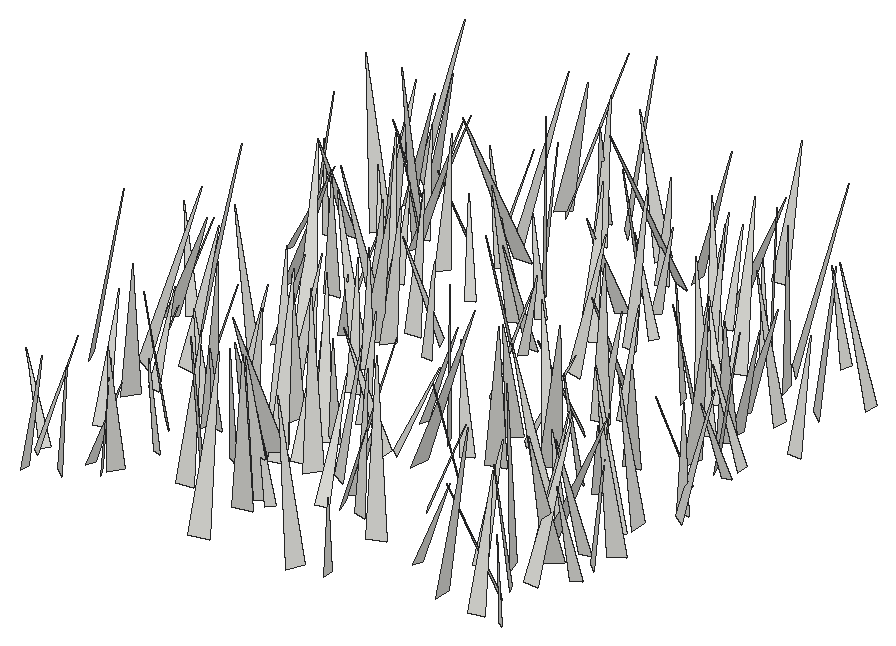
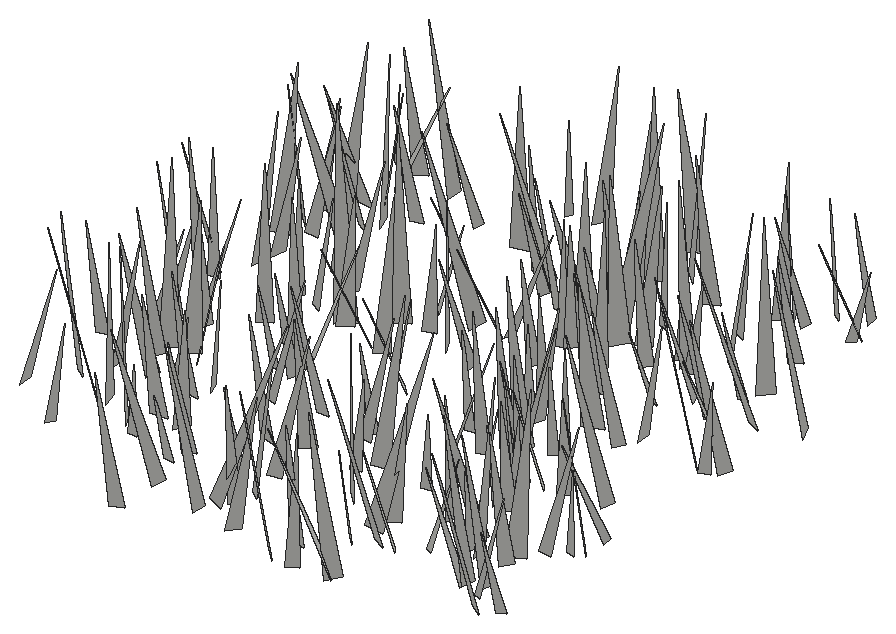
# SketchUp Ruby script. Lengths in inches.
U = 1.inch
M = Sketchup.active_model
def pt(a) = Geom::Point3d.new(a.map { |v| v * U })
def face(e, loops, mat)
  f = e.add_face(loops[0].map { |a| pt(a) })
  loops[1..].each { |l| e.add_face(l.map { |a| pt(a) }).erase! }
  f.material = f.back_material = mat if mat
  f
end
# faces: each face lists its corners as indices into pts; further lists are holes
def faces(e, pts, list, mat = nil) = list.each { |f| face(e, (f[0].is_a?(Array) ? f : [f]).map { |l| l.map { |i| pts[i] } }, mat) }
# xy, xz, yz: faces in a plane at the given z, y or x. An outline is a flat list of corners, or four numbers for a rectangle; further outlines are holes
def ring(l) = l.size == 4 ? [[l[0], l[1]], [l[2], l[1]], [l[2], l[3]], [l[0], l[3]]] : l.each_slice(2).to_a
def flat(e, list, mat, &to3) = list.each { |f| face(e, (f[0].is_a?(Array) ? f : [f]).map { |l| ring(l).map { |u, v| to3.(u, v) } }, mat) }
def xy(e, z, list, mat = nil) = flat(e, list, mat) { |x, y| [x, y, z] }
def xz(e, y, list, mat = nil) = flat(e, list, mat) { |x, z| [x, y, z] }
def yz(e, x, list, mat = nil) = flat(e, list, mat) { |y, z| [x, y, z] }
def lines(e, pts, list) = list.each { |a, b| e.add_line(pt(pts[a]), pt(pts[b])) }
# prism: a flat outline (further loops are holes) pulled along v
def prism(e, loops, v, mat = nil)
  f = face(e, loops, mat); d = Geom::Vector3d.new(v.map { |x| x * U })
  f.pushpull(f.normal.samedirection?(d) ? d.length : -d.length)
end
def box(e, o, s, mat = nil) = prism(e, [[o, [o[0] + s[0], o[1], o[2]], [o[0] + s[0], o[1] + s[1], o[2]], [o[0], o[1] + s[1], o[2]]]], [0, 0, s[2]], mat)
def at(x, y, z, deg = 0) = Geom::Transformation.translation(pt([x, y, z])) * Geom::Transformation.rotation(ORIGIN, Z_AXIS, deg.degrees)
def axes(o, x, y, z) = Geom::Transformation.new([*x, 0, *y, 0, *z, 0, *pt(o).to_a, 1])
def part(name) = M.definitions.add(name)
# library, detail: a bought-in or finely detailed component or shape, given as its bounding box
def library(name, o, s) = part(name).tap { |d| box(d.entities, o, s) }
def detail(e, o, s) = box(e.add_group.entities, o, s)
def put(e, d, t, mat = nil) = e.add_instance(d, t).tap { |i| i.material = mat if mat }
def group(e, t, mat = nil) = e.add_group.tap { |g| g.transformation = t; g.material = mat if mat }.entities
root = M.entities
c1 = part("fur_instance\#9")
p = [[0.8125,0,1.79],[0.67,-0.02,1.48],[0,-0.11,0],[0,0.11,0]]
faces(c1.entities,p,[[0,1,2,3]])
put(root,c1,axes([499.63,421.45,-21.66],[6.18065,2.99725,1.89028],[2.99834,-6.44896,0.42186],[-1.88855,-0.42956,6.85609]))
put(root,c1,axes([500.26,456.0625,-21.66],[-0.72601,3.76819,0.7458],[3.80081,0.81458,-0.41575],[0.55615,-0.64789,3.8149]))
put(root,c1,axes([501.63,430.7,-21.66],[-2.18486,3.79279,1.02862],[3.92891,2.13324,0.47945],[0.08359,-1.13179,4.35074]))
put(root,c1,axes([501.8,446.09,-21.66],[0.50374,3.60666,1.32904],[3.78488,-0.69911,0.46265],[-0.67011,-1.23747,3.61216]))
put(root,c1,axes([501.12,445.19,-21.66],[4.60486,4.04407,1.88978],[4.30358,-4.74303,-0.33665],[-1.18533,-1.50984,6.1193]))
put(root,c1,axes([501.34,428.43,-21.66],[4.04394,2.43918,0.42992],[2.39305,-4.06014,0.52577],[-0.63852,0.23141,4.69325]))
put(root,c1,axes([500.875,442.96,-21.66],[4.1398,0.29454,0.02134],[0.28882,-4.10074,0.57065],[-0.06159,0.56772,4.11084]))
put(root,c1,axes([500.51,429.625,-21.66],[5.28357,-2.5058,0.04843],[-2.504,-5.27298,0.35108],[0.10676,0.33794,5.83712]))
put(root,c1,axes([503.16,455.23,-21.66],[-1.78915,-3.44674,0.35763],[-3.41457,1.82215,0.479],[0.59044,0.09337,3.85378]))
put(root,c1,axes([503.31,447.18,-21.66],[-0.2394,-4.99537,0.47277],[-5.01072,0.21306,-0.28607],[-0.26442,0.48521,4.99291]))
put(root,c1,axes([501.99,456.89,-21.66],[3.861,5.57007,1.34937],[5.71182,-3.87341,-0.35436],[-0.47072,-1.31331,6.76812]))
put(root,c1,axes([504.5625,448.95,-21.66],[-4.39266,5.33205,2.64396],[5.82364,4.52851,0.54275],[1.2274,-2.40386,6.88706]))
put(root,c1,axes([505.53,408.68,-21.66],[-3.05082,2.35934,0.28628],[2.37608,3.01778,0.45074],[-0.05159,-0.53147,3.83025]))
put(root,c1,axes([502.97,429.98,-21.66],[5.7382,5.20942,1.87337],[5.41352,-5.84467,-0.3291],[-1.15821,-1.50876,7.74318]))
put(root,c1,axes([503.29,422.85,-21.66],[3.5873,6.66463,1.07182],[6.75002,-3.55215,-0.50434],[-0.05834,-1.18311,7.55193]))
put(root,c1,axes([503.45,453.67,-21.66],[5.71322,-0.96407,0.62556],[-0.92485,-5.73993,-0.39936],[-0.68221,-0.29224,5.7802]))
put(root,c1,axes([504.38,450.26,-21.66],[3.71133,-3.4553,1.19556],[-3.62183,-3.7076,0.52772],[-0.50083,1.20708,5.04327]))
put(root,c1,axes([505.4,407.75,-21.66],[2.99735,3.72962,0.28981],[3.68324,-3.00724,0.60693],[-0.65404,0.15682,4.74613]))
put(root,c1,axes([504.83,454.17,-21.66],[6.44965,-0.53992,1.19924],[-0.48241,-6.55498,-0.35669],[-1.22351,-0.26161,6.46237]))
put(root,c1,axes([506.6875,413.67,-21.66],[-1.85743,4.94831,0.92273],[4.99711,1.93095,-0.29602],[0.60509,-0.75691,5.27714]))
put(root,c1,axes([506.23,420.38,-21.66],[-0.0874,4.08723,0.80677],[4.1529,0.14964,-0.30818],[0.33125,-0.79758,4.07653]))
put(root,c1,axes([506.19,405.4,-21.66],[4.45017,0.43948,1.54669],[0.28501,-4.6951,0.51402],[-1.58245,0.39027,4.44218]))
put(root,c1,axes([505.49,418.73,-21.66],[5.14782,-4.26055,1.16689],[-4.27581,-5.25589,-0.32723],[-1.10966,0.4872,6.67423]))
put(root,c1,axes([504.15,438.8,-21.66],[6.51578,-0.90085,0.09034],[-0.89347,-6.50413,-0.41604],[-0.1463,-0.39981,6.56459]))
put(root,c1,axes([506.85,450.32,-21.66],[-6.68895,-1.28776,2.75903],[-1.15,7.23488,0.5888],[2.81923,-0.10417,6.78629]))
put(root,c1,axes([504.95,454.59,-21.66],[4.62251,0.92588,0.22465],[0.9419,-4.60847,-0.38752],[-0.14333,-0.42437,4.69837]))
put(root,c1,axes([506.24,424.2,-21.66],[-0.03084,5.75903,1.17934],[5.85206,0.14189,-0.53988],[0.55736,-1.17118,5.73375]))
put(root,c1,axes([508.36,429.35,-21.66],[-5.56537,0.35389,1.01892],[0.25962,5.63719,-0.53984],[1.04691,0.48332,5.55042]))
put(root,c1,axes([507.75,449.98,-21.66],[-3.18277,2.93848,0.48438],[2.88307,3.21784,-0.5768],[0.74643,0.10079,4.29324]))
put(root,c1,axes([507.6,439.44,-21.66],[1.5026,-5.2869,1.47769],[-5.48951,-1.44343,0.41772],[0.01326,1.53554,5.48039]))
put(root,c1,axes([508.65,448.72,-21.66],[-3.91635,-3.27614,1.36892],[-3.24396,4.13005,0.60351],[1.44353,0.39293,5.07017]))
put(root,c1,axes([509.24,443.92,-21.66],[3.60121,-2.60608,3.3834],[-3.59297,-4.24118,0.55747],[-2.30861,2.53545,4.41017]))
put(root,c1,axes([508.61,406.51,-21.66],[2.85129,3.39796,1.84964],[3.79237,-2.9092,-0.50161],[-0.76499,-1.75715,4.40731]))
put(root,c1,axes([510.41,441.83,-21.66],[-3.8761,2.85036,0.12124],[2.83481,3.87102,-0.37744],[0.32105,0.23257,4.79648]))
put(root,c1,axes([510.11,452.15,-21.66],[-1.91573,-3.10975,0.18965],[-3.07242,1.92263,0.49017],[0.51647,-0.09744,3.61944]))
put(root,c1,axes([510.35,416.87,-21.66],[-3.95359,-4.39819,1.62013],[-4.4402,4.19331,0.54823],[1.50116,0.81969,5.8885]))
put(root,c1,axes([509.02,422.57,-21.66],[4.30125,1.72732,0.68489],[1.69718,-4.35514,0.32517],[-0.75649,0.05042,4.6237]))
put(root,c1,axes([510.15,442.01,-21.66],[3.4021,4.35261,1.87369],[4.47593,-3.70904,0.48912],[-1.55627,-1.15238,5.50275]))
put(root,c1,axes([508.04,448.61,-21.66],[6.4862,-0.82849,0.61771],[-0.87391,-6.49276,0.46816],[-0.55158,0.54452,6.52212]))
put(root,c1,axes([510.38,443.73,-21.66],[-2.95191,2.4359,0.97471],[2.3622,3.10602,-0.60836],[1.1418,-0.12828,3.77853]))
put(root,c1,axes([509.4,439.62,-21.66],[3.16954,2.48643,0.53995],[2.54162,-3.13416,-0.48689],[-0.1185,-0.71733,3.99891]))
put(root,c1,axes([512.21,430.4,-21.66],[-3.14428,7.71271,0.49149],[7.72648,3.12546,0.38342],[-0.17032,-0.59964,8.32018]))
put(root,c1,axes([509.08,431.34,-21.66],[4.36325,-2.68491,0.18726],[-2.69098,-4.34538,0.39756],[0.04948,0.43666,5.1077]))
put(root,c1,axes([511.69,419.69,-21.66],[-3.05036,2.77962,1.08054],[2.93347,3.07501,0.37088],[0.53722,-1.00823,4.11016]))
put(root,c1,axes([511.12,424.8,-21.66],[1.03899,3.82207,0.22987],[3.79032,-1.06041,0.49963],[-0.54276,-0.08876,3.92914]))
put(root,c1,axes([509.55,408.9375,-21.66],[4.16125,-1.09144,0.28201],[-1.11074,-4.15389,0.31328],[-0.19241,0.37504,4.29058]))
put(root,c1,axes([512.47,438.875,-21.66],[-6.25427,-0.78477,1.30734],[-0.71032,6.38344,0.43371],[1.34924,-0.27711,6.28838]))
put(root,c1,axes([510.92,408.51,-21.66],[4.15437,2.45212,1.76514],[2.75663,-4.30471,-0.50784],[-1.23677,-1.35794,4.79727]))
put(root,c1,axes([511.65,447.32,-21.66],[4.3952,-2.19196,2.60814],[-2.70598,-4.83259,0.49862],[-2.06997,1.6632,4.88608]))
put(root,c1,axes([512.28,413.18,-21.66],[0.90627,3.33198,1.59944],[3.57947,-1.20149,0.47479],[-0.9207,-1.39138,3.42023]))
put(root,c1,axes([511.11,440.0625,-21.66],[3.01124,-3.84874,1.35887],[-4.04465,-3.04041,0.35153],[-0.54781,1.29229,4.87409]))
put(root,c1,axes([511.59,409.36,-21.66],[4.45698,-3.93649,1.376],[-3.92382,-4.64074,-0.56675],[-1.41173,0.47074,5.91941]))
put(root,c1,axes([512,435.36,-21.66],[1.97582,-3.11414,0.08334],[-3.10691,-1.9626,0.3224],[0.22782,0.24287,3.67393]))
put(root,c1,axes([512.125,453.625,-21.66],[3.35941,2.47012,0.56366],[2.52325,-3.34641,-0.37364],[-0.22894,-0.63632,4.15301]))
put(root,c1,axes([512.65,418.83,-21.66],[7.01983,-0.71592,2.31882],[-0.6287,-7.39114,-0.37866],[-2.34397,-0.1616,7.04608]))
put(root,c1,axes([515.92,432.38,-21.66],[-6.2227,2.39174,0.32304],[2.36421,6.22042,-0.51348],[0.48507,0.36431,6.64671]))
put(root,c1,axes([513.51,418.64,-21.66],[0.0585,-4.06465,0.78718],[-4.11626,0.02739,0.44734],[0.44434,0.78888,4.04038]))
put(root,c1,axes([514.78,450.38,-21.66],[2.55776,-3.86723,2.22173],[-4.13899,-3.01226,-0.47827],[-1.66143,1.55064,4.61182]))
put(root,c1,axes([513.74,436.98,-21.66],[3.88682,0.49651,1.01606],[0.42112,-4.01087,0.34905],[-1.04955,0.22945,3.90283]))
put(root,c1,axes([513.02,459.66,-21.66],[5.25974,-3.61511,1.15521],[-3.73911,-5.27428,0.51907],[-0.65007,1.0869,6.36116]))
put(root,c1,axes([515.29,452.08,-21.66],[-0.22294,-7.81188,0.28991],[-7.80547,0.20653,-0.4373],[-0.42917,0.30182,7.80282]))
put(root,c1,axes([513.73,453.51,-21.66],[3.6487,6.36792,1.23917],[6.47764,-3.65398,-0.29593],[-0.35515,-1.22351,7.3332]))
put(root,c1,axes([513.47,459.41,-21.66],[5.3948,4.35682,0.5893],[4.31887,-5.42625,0.57994],[-0.82254,0.08385,6.9101]))
put(root,c1,axes([514.63,426.04,-21.66],[0.44242,5.64748,1.29703],[5.78226,-0.34572,-0.46699],[0.37666,-1.32609,5.6455]))
put(root,c1,axes([516.04,445.05,-21.66],[-1.47936,3.73163,0.54523],[3.76451,1.42617,0.45319],[-0.22551,-0.67216,3.98851]))
put(root,c1,axes([515.53,454.49,-21.66],[2.40724,3.27999,1.19788],[3.2967,-2.61439,0.53362],[-1.15108,-0.62824,4.03341]))
put(root,c1,axes([514.82,420.93,-21.66],[3.66382,-3.28739,1.57998],[-3.52995,-3.75957,0.36325],[-0.918,1.33625,4.90903]))
put(root,c1,axes([514.3125,435.91,-21.66],[4.31409,-4.88001,1.43702],[-5.06352,-4.30068,0.59646],[-0.49016,1.47666,6.48614]))
put(root,c1,axes([515.33,436.38,-21.66],[-4.36102,2.95909,2.58691],[3.11538,4.95832,-0.41976],[2.39639,-1.06094,5.25343]))
put(root,c1,axes([516.44,432.55,-21.66],[-4.17339,1.81444,1.20525],[1.74242,4.34394,-0.50613],[1.30721,0.0026,4.52253]))
put(root,c1,axes([515.98,438.43,-21.66],[-1.18817,5.57554,2.26119],[5.96275,1.39894,-0.31626],[0.80332,-2.13721,5.69196]))
put(root,c1,axes([518.3,438.93,-21.66],[-4.34148,-1.68145,0.56308],[-1.64517,4.37512,0.38015],[0.66161,-0.1544,4.64018]))
put(root,c1,axes([516.375,460.26,-21.66],[1.54796,-4.76639,0.70367],[-4.81569,-1.50748,0.38266],[0.1508,0.78667,4.99682]))
put(root,c1,axes([517.9375,429.02,-21.66],[-0.91047,5.0165,1.03079],[5.11456,0.83694,0.44447],[-0.2628,-1.09133,5.07905]))
put(root,c1,axes([516.94,410.7,-21.66],[-1.46748,5.77462,2.34569],[6.13429,1.76496,-0.50731],[1.10405,-2.13089,5.93652]))
put(root,c1,axes([517.21,423.36,-21.66],[5.69628,-2.00129,2.37758],[-1.98509,-6.1627,-0.4314],[-2.39112,0.34864,6.02217]))
put(root,c1,axes([517.49,415.62,-21.66],[-2.05605,-4.2865,1.82271],[-4.5186,2.31917,0.35698],[1.13077,1.47345,4.74068]))
put(root,c1,axes([516.99,418.56,-21.66],[3.45501,-4.88886,0.26504],[-4.85303,-3.46254,-0.60598],[-0.64754,-0.13474,5.95575]))
put(root,c1,axes([518.24,457.41,-21.66],[-0.17119,5.69768,1.30234],[5.83131,0.07859,0.42267],[-0.39436,-1.31119,5.68456]))
put(root,c1,axes([518.46,419.55,-21.66],[-5.59489,5.13542,2.2708],[5.22691,5.9344,-0.54239],[2.05147,-1.11455,7.57503]))
put(root,c1,axes([518.95,423.23,-21.66],[-3.597,-0.64897,1.74683],[-0.97146,3.89365,-0.55385],[1.59023,0.91068,3.61287]))
put(root,c1,axes([518.89,436.38,-21.66],[0.06663,3.86387,1.64805],[4.18879,0.06273,-0.31643],[0.31563,-1.6482,3.85147]))
put(root,c1,axes([519.43,449.48,-21.66],[4.46233,4.90899,2.88894],[5.22756,-4.98695,0.39938],[-2.26203,-1.84084,6.62202]))
put(root,c1,axes([518.79,459.83,-21.66],[4.76999,5.26227,1.90717],[5.37132,-5.00824,0.38463],[-1.57405,-1.14351,7.09199]))
put(root,c1,axes([520.09,417.51,-21.66],[-1.2461,7.24945,1.28302],[7.36015,1.19663,0.38699],[-0.1701,-1.32928,7.34558]))
put(root,c1,axes([520.79,422.01,-21.66],[-4.49131,4.50007,0.95246],[4.50728,4.57122,-0.34355],[0.91773,-0.42777,6.34858]))
put(root,c1,axes([520.58,408.52,-21.66],[3.92843,5.06138,3.38638],[5.5366,-4.64662,0.52215],[-2.53598,-2.30413,6.38572]))
put(root,c1,axes([519.85,418,-21.66],[2.00321,-7.73932,0.37509],[-7.71802,-2.02729,-0.61059],[-0.68548,0.20889,7.97102]))
put(root,c1,axes([520.65,444.66,-21.66],[2.01145,-6.31603,1.30369],[-6.40118,-2.12156,-0.40211],[-0.78536,1.11557,6.61638]))
put(root,c1,axes([521.14,418.45,-21.66],[-1.57636,3.66287,0.67143],[3.67727,1.64614,-0.34684],[0.58749,-0.47537,3.97256]))
put(root,c1,axes([521.75,446.1,-21.66],[-1.38179,3.78074,1.32931],[4.00762,1.30133,0.46468],[-0.00636,-1.40818,3.99842]))
put(root,c1,axes([521.38,425.9,-21.66],[2.89571,-2.97183,2.13904],[-3.49598,-3.05481,0.48854],[-1.08874,1.90494,4.12046]))
put(root,c1,axes([521.46,422.47,-21.66],[0.51611,-4.80053,1.29544],[-4.96034,-0.40702,0.46794],[0.34389,1.33374,4.80546]))
put(root,c1,axes([523.24,458.54,-21.66],[-5.24229,2.67543,1.59997],[2.88849,5.34612,0.52444],[1.17239,-1.20849,5.86212]))
put(root,c1,axes([523.01,418.05,-21.66],[-6.12251,3.37612,2.03098],[3.42132,6.417,-0.35327],[1.95387,-0.65732,6.98272]))
put(root,c1,axes([522.54,405.29,-21.66],[-2.30774,6.81626,2.09214],[7.04491,2.51871,-0.43516],[1.09893,-1.8327,7.18315]))
put(root,c1,axes([522.82,412.42,-21.66],[2.11565,-6.08651,1.80009],[-6.2822,-2.27872,-0.32139],[-0.90548,1.58863,6.43571]))
put(root,c1,axes([523.21,441.02,-21.66],[-3.17607,-4.40082,1.193],[-4.40846,3.33508,0.56622],[1.16445,0.62283,5.3976]))
put(root,c1,axes([523.72,412.16,-21.66],[1.42768,-3.34431,1.65268],[-3.54003,-1.77266,-0.52903],[-1.17641,1.27565,3.59761]))
put(root,c1,axes([522.42,410.53,-21.66],[2.16747,-6.96935,1.82134],[-7.20329,-2.08612,0.58967],[0.04123,1.91397,7.27476]))
put(root,c1,axes([524.07,442.1875,-21.66],[-0.19346,-4.85951,0.89963],[-4.92735,0.1202,-0.41034],[-0.38132,0.91231,4.84602]))
put(root,c1,axes([525.48,423.48,-21.66],[-5.10669,0.68056,0.36828],[0.71376,5.09217,0.48729],[0.29888,-0.53268,5.12875]))
put(root,c1,axes([524.06,441.12,-21.66],[3.08181,-1.73974,0.98019],[-1.88437,-3.1302,0.36886],[-0.66077,0.81254,3.51969]))
put(root,c1,axes([525.2,453.6,-21.66],[-3.25628,-4.53556,1.56998],[-4.60157,3.48952,0.53691],[1.36443,0.94415,5.55755]))
put(root,c1,axes([526.71,456.3,-21.66],[-3.06964,-6.81398,0.3454],[-6.81954,3.05272,-0.38339],[-0.20825,0.47214,7.46364]))
put(root,c1,axes([525.09,418.38,-21.66],[2.3418,4.95634,1.60959],[5.19702,-2.35112,-0.32146],[-0.38351,-1.59595,5.4723]))
put(root,c1,axes([525.81,450.5625,-21.66],[1.38462,-5.25865,0.1546],[-5.22749,-1.39323,-0.57157],[-0.5921,0.00308,5.40776]))
put(root,c1,axes([524.69,428.875,-21.66],[4.46137,-0.22154,0.62784],[-0.29219,-4.4737,0.49769],[-0.59824,0.53291,4.43905]))
put(root,c1,axes([525.53,455.53,-21.66],[2.1664,-3.98299,1.68795],[-4.30586,-2.16689,0.41322],[-0.41582,1.68731,4.51516]))
put(root,c1,axes([526.5625,445.68,-21.66],[-2.92394,5.35838,1.35906],[5.44647,3.05552,-0.32925],[0.94614,-1.02969,6.09534]))
put(root,c1,axes([526.66,414.47,-21.66],[-2.17484,4.53028,0.06229],[4.50087,2.16823,-0.54601],[0.51907,0.1805,4.99552]))
put(root,c1,axes([526.32,434.56,-21.66],[3.1839,3.43631,0.24845],[3.39454,-3.18669,0.57383],[-0.5891,0.20968,4.64932]))
put(root,c1,axes([525.89,423.99,-21.66],[2.47782,3.1575,0.0552],[3.13992,-2.45577,-0.47176],[0.33732,-0.3344,3.98583]))
put(root,c1,axes([527.96,427.76,-21.66],[5.01686,3.02729,2.73746],[3.17963,-5.61852,0.38618],[-2.55892,-1.04628,5.84673]))
put(root,c1,axes([527.83,452.02,-21.66],[3.18405,-1.52738,1.26596],[-1.78098,-3.25535,0.55182],[-0.87386,1.06936,3.48806]))
put(root,c1,axes([527.39,417.14,-21.66],[3.65064,-1.60023,0.53489],[-1.66152,-3.63138,0.47591],[-0.29361,0.65299,3.95745]))
put(root,c1,axes([530.08,448.92,-21.66],[-3.96056,0.86775,0.15545],[0.85071,3.94968,-0.37345],[0.23119,0.33194,4.03727]))
put(root,c1,axes([527.08,457.82,-21.66],[6.44978,-0.00096,0.92482],[0.04605,-6.50733,-0.32793],[-0.92367,-0.33115,6.44144]))
put(root,c1,axes([529.59,446.68,-21.66],[0.8824,6.11345,1.2337],[6.18895,-1.01221,0.58924],[-0.77016,-1.12963,6.14863]))
put(root,c1,axes([527.76,415.58,-21.66],[6.78168,2.91502,1.19431],[2.8839,-6.88568,0.43057],[-1.26762,-0.07012,7.36906]))
put(root,c1,axes([528.84,441.17,-21.66],[0.94432,5.62245,1.27282],[5.76049,-0.87093,-0.42662],[0.22085,-1.32412,5.68522]))
put(root,c1,axes([529.69,415.08,-21.66],[1.56528,5.39191,1.82425],[5.61252,-1.77733,0.43748],[-0.9488,-1.61836,5.59744]))
put(root,c1,axes([530.79,406.22,-21.66],[-6.02179,2.8816,2.13168],[3.11245,6.27078,0.31555],[1.77772,-1.21792,6.66828]))
put(root,c1,axes([530.41,426.75,-21.66],[1.59272,-3.9303,2.28796],[-4.37909,-1.9795,-0.352],[-1.22702,1.96293,4.22612]))
put(root,c1,axes([528.25,423.85,-21.66],[7.76844,-0.71206,0.72464],[-0.74639,-7.79129,0.34557],[-0.68922,0.41169,7.79335]))
put(root,c1,axes([531.84,423.93,-21.66],[-3.00946,-2.45302,0.73779],[-2.54129,3.00205,-0.38468],[0.32167,0.76736,3.86344]))
put(root,c1,axes([531.17,431.29,-21.66],[3.50702,-4.68842,0.88051],[-4.69288,-3.58696,-0.4079],[-0.85643,0.45629,5.84073]))
put(root,c1,axes([532.91,413,-21.66],[-2.11891,6.73628,2.3501],[7.12334,2.13432,0.30482],[0.39806,-2.33612,7.05509]))
put(root,c1,axes([531.97,461.18,-21.66],[-1.06035,5.5551,1.84187],[5.77115,1.30347,-0.60889],[0.97234,-1.67863,5.62252]))
put(root,c1,axes([532.98,441.95,-21.66],[-1.82356,-4.42835,0.39133],[-4.41286,1.85435,0.42054],[0.53859,0.19978,4.77062]))
put(root,c1,axes([533.375,453.39,-21.66],[-0.09668,3.9627,0.07364],[3.92699,0.08582,0.53775],[-0.5359,-0.08606,3.92724]))
put(root,c1,axes([532.85,451.67,-21.66],[-1.4542,4.67664,1.33998],[4.76533,1.65076,-0.58976],[0.97884,-1.08869,4.86188]))
put(root,c1,axes([533.3,406.875,-21.66],[3.51099,-0.42801,1.09439],[-0.295,-3.65871,-0.48452],[-1.13748,-0.37227,3.50364]))
put(root,c1,axes([534.71,434.94,-21.66],[-3.28468,-3.33783,0.1825],[-3.30088,3.27904,0.56182],[0.52783,-0.26523,4.64915]))
put(root,c1,axes([533.04,418.79,-21.66],[3.15167,2.15202,0.19961],[2.1362,-3.1554,0.29004],[-0.32814,0.12762,3.80527]))
put(root,c1,axes([532.47,430.95,-21.66],[3.00056,3.161,0.00616],[3.13284,-2.97269,-0.58633],[0.42105,-0.40809,4.31874]))
put(root,c1,axes([531.8,456.5625,-21.66],[5.92157,-1.3609,0.111],[-1.36516,-5.91048,0.36315],[-0.02664,0.3788,6.06507]))
put(root,c1,axes([532.87,426.97,-21.66],[3.4393,-6.56896,1.063],[-6.65437,-3.3911,0.57422],[0.02233,1.20797,7.39258]))
put(root,c1,axes([535.6,449.12,-21.66],[-5.07407,3.61415,0.85454],[3.5922,5.14344,-0.42375],[0.94256,-0.14624,6.2152]))
put(root,c1,axes([533.98,438.07,-21.66],[3.92282,-1.4058,1.44453],[-1.66907,-4.03753,0.60333],[-1.1301,1.0833,4.1232]))
put(root,c1,axes([535.75,429.85,-21.66],[2.97491,-4.25566,3.74848],[-5.0806,-3.88069,-0.37363],[-2.51977,2.80026,5.17891]))
put(root,c1,axes([534.66,436.96,-21.66],[-1.49682,6.02983,3.22428],[6.74332,1.8484,-0.32627],[1.1325,-3.03643,6.20426]))
put(root,c1,axes([535.79,437.98,-21.66],[0.78964,4.34465,0.57519],[4.335,-0.86018,0.54605],[-0.64386,-0.46311,4.38193]))
put(root,c1,axes([537.44,443.09,-21.66],[-4.30965,-1.39305,1.63599],[-1.58025,4.5392,-0.29767],[1.45598,0.80324,4.51941]))
put(root,c1,axes([538.45,425.7,-21.66],[-6.00997,1.04438,1.22572],[1.13938,6.10462,0.38513],[1.13796,-0.59647,6.08787]))
put(root,c1,axes([537.79,452.15,-21.66],[-0.46969,3.55211,0.73396],[3.59032,0.35011,0.60316],[-0.51554,-0.79795,3.53189]))
put(root,c1,axes([538.04,448.76,-21.66],[-1.0825,6.58238,0.66021],[6.6005,1.02978,0.55528],[-0.44383,-0.73975,6.64764]))
put(root,c1,axes([538.19,444.93,-21.66],[-0.0106,6.43156,0.96228],[6.47441,-0.07994,0.60561],[-0.61077,-0.95901,6.403]))
put(root,c1,axes([536,429.49,-21.66],[5.23004,-6.31048,0.45418],[-6.32662,-5.22094,0.31214],[-0.04891,0.54893,8.19012]))
put(root,c1,axes([539.91,444.24,-21.66],[-2.40389,3.30252,0.08348],[3.28439,2.37806,0.4999],[-0.35549,-0.36124,4.05406]))
put(root,c1,axes([539.24,428.98,-21.66],[1.51862,3.68557,2.40948],[4.21899,-1.94756,0.31991],[-1.2606,-2.07817,3.97332]))
put(root,c1,axes([537.43,412.21,-21.66],[4.04534,-0.8517,0.30361],[-0.87788,-4.03293,0.38361],[-0.21657,0.43867,4.11619]))
put(root,c1,axes([539.35,450.86,-21.66],[5.6621,3.46946,2.68851],[3.90579,-5.98471,-0.5026],[-2.00251,-1.86297,6.62147]))
put(root,c1,axes([540.9375,440.56,-21.66],[-4.28874,-2.62611,1.19653],[-2.76089,4.3576,-0.33198],[0.84,0.91449,5.01792]))
put(root,c1,axes([541.32,423.95,-21.66],[1.53479,-3.08573,1.52348],[-3.30012,-1.79268,-0.30636],[-0.97569,1.2095,3.43271]))
put(root,c1,axes([541.95,440.05,-21.66],[-4.3858,5.26104,2.02142],[5.54364,4.48874,0.34523],[1.01623,-1.78118,6.84066]))
put(root,c1,axes([541.33,414.58,-21.66],[-0.63443,5.02312,1.44392],[5.17666,0.80438,-0.52377],[0.72032,-1.3566,5.03586]))
put(root,c1,axes([540.72,433.05,-21.66],[2.46673,-5.38252,0.46134],[-5.39282,-2.42347,0.55987],[0.31917,0.65147,5.89431]))
put(root,c1,axes([542.3,449.09,-21.66],[5.88559,1.89129,2.87248],[1.95642,-6.52369,0.2867],[-2.82853,-0.57687,6.17535]))
put(root,c1,axes([541.33,428.39,-21.66],[1.84889,-3.8875,0.07331],[-3.87281,-1.83403,0.41727],[0.34554,0.24513,4.2845]))
put(root,c1,axes([541.73,409.71,-21.66],[7.00703,0.38351,2.14023],[0.30488,-7.32356,0.31416],[-2.15283,0.21111,7.01048]))
put(root,c1,axes([543.16,416.17,-21.66],[-6.66859,-2.01923,2.71074],[-2.32845,7.09045,-0.44648],[2.45024,1.24248,6.95328]))
put(root,c1,axes([541.03,451.59,-21.66],[5.81873,5.70667,1.51485],[5.84557,-5.86726,-0.35074],[-0.83073,-1.31442,8.14252]))
put(root,c1,axes([543.62,454.43,-21.66],[-3.82053,1.38738,1.41647],[1.59253,3.97908,0.39802],[1.18113,-0.87734,4.0451]))
put(root,c1,axes([545.35,412.03,-21.66],[-3.79986,-3.34827,0.10157],[-3.34083,3.7767,-0.4853],[-0.24505,0.43103,5.04126]))
put(root,c1,axes([545.16,444.76,-21.66],[-5.94659,0.26274,1.16381],[0.1992,6.05181,-0.34844],[1.17635,0.30341,5.94219]))
put(root,c1,axes([542.13,444.33,-21.66],[5.3173,-1.56529,0.48292],[-1.59322,-5.32309,0.28875],[-0.38078,0.41424,5.53538]))
put(root,c1,axes([545.08,413.49,-21.66],[-4.18009,-2.38384,1.39005],[-2.61185,4.23208,-0.59649],[0.8906,1.22265,4.77494]))
put(root,c1,axes([543.9,417.67,-21.66],[2.83544,5.2975,1.05869],[5.3487,-2.92083,0.29014],[-0.75876,-0.79328,6.00159]))
put(root,c1,axes([546.26,424.5625,-21.66],[-6.22467,1.67352,0.58559],[1.62437,6.23957,-0.56507],[0.71064,0.39649,6.42089]))
put(root,c1,axes([545.46,434,-21.66],[-2.21382,-3.77344,0.32599],[-3.76288,2.23425,0.30817],[0.43109,0.1241,4.36404]))
put(root,c1,axes([543.75,436.35,-21.66],[6.97924,-1.80721,1.76653],[-1.77915,-7.19853,-0.33521],[-1.79479,0.10824,7.20163]))
put(root,c1,axes([543.86,440.26,-21.66],[3.44417,-6.15496,0.43731],[-6.17002,-3.42915,0.33004],[0.07525,0.54268,7.04535]))
put(root,c1,axes([543.71,441.61,-21.66],[5.53978,-0.90724,0.62547],[-0.85463,-5.56113,-0.49688],[-0.69563,-0.39269,5.59154]))
put(root,c1,axes([545.49,408.95,-21.66],[-2.00411,5.21831,1.67163],[5.38658,2.20263,-0.41796],[1.00489,-1.39973,5.57427]))
put(root,c1,axes([546.15,420.79,-21.66],[0.08099,-5.17118,1.20761],[-5.27072,-0.22549,-0.61212],[-0.64729,1.18913,5.13546]))
put(root,c1,axes([545.11,418.52,-21.66],[3.26606,-6.16963,0.62937],[-6.14796,-3.31446,-0.58694],[-0.81426,0.27855,6.95607]))
put(root,c1,axes([543.04,420.59,-21.66],[6.75875,-1.16964,0.00047],[-1.16859,-6.75255,0.29358],[0.0496,0.28936,6.85293]))
put(root,c1,axes([545.83,414.93,-21.66],[0.77683,6.56918,0.32302],[6.56801,-0.79193,0.30978],[-0.34589,-0.28401,6.60769]))
put(root,c1,axes([547.17,437.86,-21.66],[-4.29082,0.07848,0.62907],[0.12494,4.3243,0.31276],[0.62151,-0.32753,4.28013]))
put(root,c1,axes([546.57,426.47,-21.66],[5.59524,-0.57904,3.08549],[-0.36766,-6.38318,-0.53118],[-3.11775,-0.28642,5.59999]))
put(root,c1,axes([545.68,436.68,-21.66],[5.68987,2.39384,1.65752],[2.61602,-5.80047,-0.60296],[-1.2784,-1.21517,6.14342]))
put(root,c1,axes([547.16,436.09,-21.66],[0.58704,-3.79537,0.45103],[-3.78334,-0.64184,-0.47675],[-0.5428,0.36891,3.81079]))
put(root,c1,axes([548.85,450.76,-21.66],[-5.68888,-0.08485,0.69236],[-0.12916,5.71868,-0.36046],[0.68548,0.37338,5.67808]))
put(root,c1,axes([546.47,447.39,-21.66],[-3.30417,-4.76212,3.2823],[-5.25525,4.05058,0.5865],[2.41528,2.29867,5.7664]))
put(root,c1,axes([547.79,408.87,-21.66],[1.56672,2.93333,1.48069],[3.11219,-1.85095,0.37383],[-1.05412,-1.105,3.30444]))
put(root,c1,axes([547.71,419.7,-21.66],[3.73887,4.62596,1.90486],[4.75099,-4.02818,0.45718],[-1.5672,-1.17533,5.9304]))
put(root,c1,axes([548.09,417.35,-21.66],[1.30026,-4.12004,1.09762],[-4.18224,-1.45572,-0.50983],[-0.82967,0.8811,4.29016]))
put(root,c1,axes([548.19,421.96,-21.66],[-2.64442,5.36733,3.49605],[6.32318,2.79183,0.49668],[1.02376,-3.3795,5.96276]))
put(root,c1,axes([547.81,430.08,-21.66],[0.13174,-4.85064,1.64659],[-5.10405,0.01535,0.4536],[0.43432,1.65178,4.83118]))
put(root,c1,axes([548.88,441.76,-21.66],[-0.27729,4.76979,1.49646],[4.98187,0.38774,-0.31274],[0.41383,-1.47171,4.7676]))
put(root,c1,axes([548.24,429.13,-21.66],[2.85218,4.71528,1.10181],[4.83661,-2.83604,-0.38317],[-0.23454,-1.14272,5.49745]))
